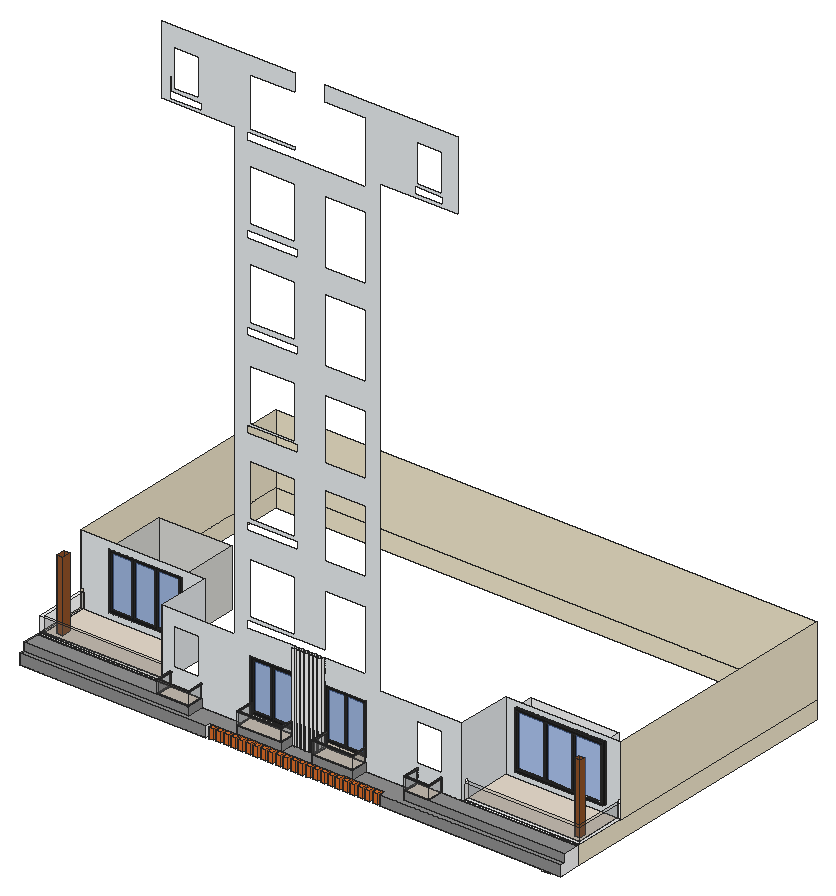
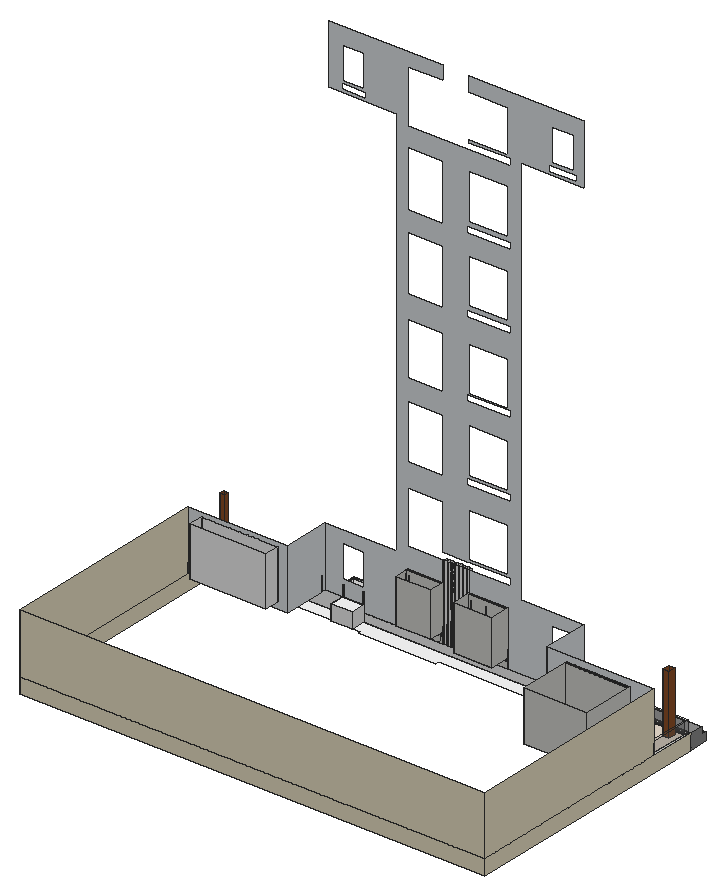
# SketchUp Ruby script. Lengths in inches.
U = 1.inch
M = Sketchup.active_model
def pt(a) = Geom::Point3d.new(a.map { |v| v * U })
def face(e, loops, mat)
  f = e.add_face(loops[0].map { |a| pt(a) })
  loops[1..].each { |l| e.add_face(l.map { |a| pt(a) }).erase! }
  f.material = f.back_material = mat if mat
  f
end
# faces: each face lists its corners as indices into pts; further lists are holes
def faces(e, pts, list, mat = nil) = list.each { |f| face(e, (f[0].is_a?(Array) ? f : [f]).map { |l| l.map { |i| pts[i] } }, mat) }
# xy, xz, yz: faces in a plane at the given z, y or x. An outline is a flat list of corners, or four numbers for a rectangle; further outlines are holes
def ring(l) = l.size == 4 ? [[l[0], l[1]], [l[2], l[1]], [l[2], l[3]], [l[0], l[3]]] : l.each_slice(2).to_a
def flat(e, list, mat, &to3) = list.each { |f| face(e, (f[0].is_a?(Array) ? f : [f]).map { |l| ring(l).map { |u, v| to3.(u, v) } }, mat) }
def xy(e, z, list, mat = nil) = flat(e, list, mat) { |x, y| [x, y, z] }
def xz(e, y, list, mat = nil) = flat(e, list, mat) { |x, z| [x, y, z] }
def yz(e, x, list, mat = nil) = flat(e, list, mat) { |y, z| [x, y, z] }
def lines(e, pts, list) = list.each { |a, b| e.add_line(pt(pts[a]), pt(pts[b])) }
# prism: a flat outline (further loops are holes) pulled along v
def prism(e, loops, v, mat = nil)
  f = face(e, loops, mat); d = Geom::Vector3d.new(v.map { |x| x * U })
  f.pushpull(f.normal.samedirection?(d) ? d.length : -d.length)
end
def box(e, o, s, mat = nil) = prism(e, [[o, [o[0] + s[0], o[1], o[2]], [o[0] + s[0], o[1] + s[1], o[2]], [o[0], o[1] + s[1], o[2]]]], [0, 0, s[2]], mat)
def at(x, y, z, deg = 0) = Geom::Transformation.translation(pt([x, y, z])) * Geom::Transformation.rotation(ORIGIN, Z_AXIS, deg.degrees)
def axes(o, x, y, z) = Geom::Transformation.new([*x, 0, *y, 0, *z, 0, *pt(o).to_a, 1])
def part(name) = M.definitions.add(name)
# library, detail: a bought-in or finely detailed component or shape, given as its bounding box
def library(name, o, s) = part(name).tap { |d| box(d.entities, o, s) }
def detail(e, o, s) = box(e.add_group.entities, o, s)
def put(e, d, t, mat = nil) = e.add_instance(d, t).tap { |i| i.material = mat if mat }
def group(e, t, mat = nil) = e.add_group.tap { |g| g.transformation = t; g.material = mat if mat }.entities
root = M.entities
M.materials.add("Generic").color = [146, 146, 146]
M.materials.add("Generic\#3").color = [226, 112, 41]
M.materials.add("Generic\#4").color = [237, 241, 244]
M.materials.add("Generic\#5").color = [249, 239, 211]
M.materials.add("Generic\#7").color = [232, 220, 205]
M.materials.add("[Color M00]").color = [255, 255, 255]
M.materials.add("[Color M06]").color = [86, 86, 86]
M.materials.add("[Color M08]").color = [30, 30, 30]
M.materials.add("[Translucent Glass Blue]1").color = [100, 149, 237]
M.materials["[Translucent Glass Blue]1"].alpha = 0.5
M.materials.add("[Translucent Glass Gray]").color = [119, 119, 119]
M.materials["[Translucent Glass Gray]"].alpha = 0.16
M.materials.add("[Wood Cherry Original]").color = [150, 85, 41]
M.materials.add("[Wood Cherry Original]1").color = [152, 86, 42]
c1 = part("Group\#10")
xy(c1.entities,0,[[0,0,98.1875,6]],"[Color M08]")
xy(c1.entities,5.79,[[5.79,0,46.2,3],[51.99,0,92.4,3]],"[Color M08]")
xy(c1.entities,117.02,[[5.79,0,46.2,3],[51.99,0,92.4,3]],"[Color M08]")
xy(c1.entities,122.8125,[[0,0,98.1875,6]],"[Color M08]")
xz(c1.entities,0,[[[0,0,98.1875,122.8125],[5.79,5.79,46.2,117.02],[51.99,5.79,92.4,117.02]]],"[Color M08]")
xz(c1.entities,3,[[5.79,5.79,46.2,117.02],[51.99,5.79,92.4,117.02]],"[Translucent Glass Blue]1")
xz(c1.entities,6,[[0,0,98.1875,122.8125]])
yz(c1.entities,0,[[0,0,6,122.8125]],"[Color M08]")
yz(c1.entities,5.79,[[0,5.79,3,117.02]],"[Color M08]")
yz(c1.entities,46.2,[[0,5.79,3,117.02]],"[Color M08]")
yz(c1.entities,51.99,[[0,5.79,3,117.02]],"[Color M08]")
yz(c1.entities,92.4,[[0,5.79,3,117.02]],"[Color M08]")
yz(c1.entities,98.1875,[[0,0,6,122.8125]],"[Color M08]")
c2 = part("Group\#11")
xy(c2.entities,0,[[0,0,175.8125,6]],"[Color M08]")
xy(c2.entities,7.33,[[7.33,0,56.16,3],[63.49,0,112.32,3],[119.65,0,168.48,3]],"[Color M08]")
xy(c2.entities,131.1,[[7.33,0,56.16,3],[63.49,0,112.32,3],[119.65,0,168.48,3]],"[Color M08]")
xy(c2.entities,138.4375,[[0,0,175.8125,6]],"[Color M08]")
xz(c2.entities,0,[[[0,0,175.8125,0,175.8125,131.1,168.48,131.1,168.48,7.33,119.65,7.33,119.65,131.1,175.8125,131.1,175.8125,138.4375,0,138.4375],[7.33,7.33,56.16,131.1],[63.49,7.33,112.32,131.1]]],"[Color M08]")
xz(c2.entities,3,[[7.33,7.33,56.16,131.1],[63.49,7.33,112.32,131.1],[119.65,7.33,168.48,131.1]],"[Translucent Glass Blue]1")
xz(c2.entities,6,[[0,0,175.8125,138.4375]])
yz(c2.entities,0,[[0,0,6,138.4375]],"[Color M08]")
yz(c2.entities,7.33,[[0,7.33,3,131.1]],"[Color M08]")
yz(c2.entities,56.16,[[0,7.33,3,131.1]],"[Color M08]")
yz(c2.entities,63.49,[[0,7.33,3,131.1]],"[Color M08]")
yz(c2.entities,112.32,[[0,7.33,3,131.1]],"[Color M08]")
yz(c2.entities,119.65,[[0,7.33,3,131.1]],"[Color M08]")
yz(c2.entities,168.48,[[0,7.33,3,131.1]],"[Color M08]")
yz(c2.entities,175.8125,[[0,0,6,138.4375]],"[Color M08]")
c3 = part("Group\#12")
xy(c3.entities,0,[[0,0,212.5625,7]],"[Color M08]")
xy(c3.entities,6.29,[[6.29,0,68.76,4],[75.05,0,137.52,4],[143.8,0,206.27,4]],"[Color M08]")
xy(c3.entities,131.21,[[6.29,0,68.76,4],[75.05,0,137.52,4],[143.8,0,206.27,4]],"[Color M08]")
xy(c3.entities,137.5,[[0,0,212.5625,7]],"[Color M08]")
xz(c3.entities,0,[[0,0,212.5625,6.29],[0,6.29,6.29,131.21],[68.76,6.29,75.05,131.21],[137.52,6.29,143.8,131.21],[206.27,6.29,212.5625,131.21],
  [0,131.21,212.5625,137.5]],"[Color M08]")
xz(c3.entities,4,[[6.29,6.29,68.76,131.21],[75.05,6.29,137.52,131.21],[143.8,6.29,206.27,131.21]],"[Translucent Glass Blue]1")
xz(c3.entities,7,[[0,0,212.5625,137.5]],"[Color M00]")
yz(c3.entities,0,[[0,0,7,137.5]],"[Color M08]")
yz(c3.entities,6.29,[[0,6.29,4,131.21]],"[Color M08]")
yz(c3.entities,68.76,[[0,6.29,4,131.21]],"[Color M08]")
yz(c3.entities,75.05,[[0,6.29,4,131.21]],"[Color M08]")
yz(c3.entities,137.52,[[0,6.29,4,131.21]],"[Color M08]")
yz(c3.entities,143.8,[[0,6.29,4,131.21]],"[Color M08]")
yz(c3.entities,206.27,[[0,6.29,4,131.21]],"[Color M08]")
yz(c3.entities,212.5625,[[0,0,7,137.5]],"[Color M08]")
xy(root,378.75,[[1471.55,257.9375,1493.05,261.625],[233.49,313.625,249.12,318.23]])
xy(root,378.75,[[209.5,261.625,209.5,313.625,233.49,313.625,233.49,296.48,249.12,296.48,249.12,313.625,509.5,313.625,509.5,261.625],[233.49,296.48,249.12,313.625]],"Generic")
xy(root,378.75,[[663.6,261.625,675.6,273.75],[681.6,261.625,693.6,273.75],[699.6,261.625,711.6,273.75],[717.6,261.625,729.6,273.75],[735.6,261.625,747.6,273.75],
  [753.6,261.625,765.6,273.75],[771.6,261.625,783.6,273.75],[789.6,261.625,801.6,273.75],[807.6,261.625,819.6,273.75],[825.6,261.625,837.6,273.75],
  [843.6,261.625,855.6,273.75],[861.6,261.625,873.6,273.75],[879.6,261.625,891.6,273.75],[897.6,261.625,909.6,273.75],[915.6,261.625,927.6,273.75],
  [933.6,261.625,945.6,273.75],[951.6,261.625,963.6,273.75],[969.6,261.625,981.6,273.75],[987.6,261.625,999.6,273.75],[1005.6,261.625,1017.6,273.75],
  [1023.6,261.625,1035.6,273.75],[1041.6,261.625,1053.6,273.75],[1059.6,261.625,1071.6,273.75]],"Generic\#3")
xy(root,378.75,[[509.5,261.625,509.5,313.625,1513,313.625,1513,261.625,1493.05,261.625,1493.05,285.22,1471.55,285.22,1471.55,261.625,1077.6,261.625,1077.6,273.75,657.6,273.75,657.6,261.625],[209.5,313.625,209.5,351.125,509.5,351.125,509.5,313.625,249.12,313.625,249.12,318.23,233.49,318.23,233.49,313.625],[509.5,313.625,509.5,360,548.8125,360,548.8125,351.125,886.67,351.125,886.67,360,1103.86,360,1103.86,351.125,1125.09,351.125,1125.09,313.625],[1125.09,313.625,1185.84,351.125],[1185.84,313.625,1513,351.125],
  [1125.09,351.125,1185.84,353.5]],"[Color M00]")
xy(root,403.0625,[[529.46,273.75,607.09,313.625],[722.84,273.75,830.21,313.625],[903.71,273.75,1001.9,313.625]])
xy(root,403.0625,[[209.5,261.625,657.6,261.625,657.6,273.75,722.84,273.75,722.84,313.625,607.09,313.625,607.09,273.75,209.5,273.75],[1077.6,261.625,1513,261.625,1513,273.75,1125.09,273.75,1125.09,313.625,1001.9,313.625,1001.9,273.75,1077.6,273.75],[830.21,273.75,903.71,273.75,903.71,313.625,901.15,313.625,901.15,305.3125,893.21,305.3125,893.21,313.625,890.65,313.625,890.65,305.3125,882.71,305.3125,882.71,313.625,880.15,313.625,880.15,305.3125,872.21,305.3125,872.21,313.625,869.65,313.625,869.65,305.3125,861.71,305.3125,861.71,313.625,859.15,313.625,859.15,305.3125,851.21,305.3125,851.21,313.625,848.65,313.625,848.65,305.3125,840.71,305.3125,840.71,313.625,838.15,313.625,838.15,305.3125,830.21,305.3125]],"Generic")
xy(root,403.0625,[[663.6,261.625,675.6,273.75],[681.6,261.625,693.6,273.75],[699.6,261.625,711.6,273.75],[717.6,261.625,729.6,273.75],[735.6,261.625,747.6,273.75],
  [753.6,261.625,765.6,273.75],[771.6,261.625,783.6,273.75],[789.6,261.625,801.6,273.75],[807.6,261.625,819.6,273.75],[825.6,261.625,837.6,273.75],
  [843.6,261.625,855.6,273.75],[861.6,261.625,873.6,273.75],[879.6,261.625,891.6,273.75],[897.6,261.625,909.6,273.75],[915.6,261.625,927.6,273.75],
  [933.6,261.625,945.6,273.75],[951.6,261.625,963.6,273.75],[969.6,261.625,981.6,273.75],[987.6,261.625,999.6,273.75],[1005.6,261.625,1017.6,273.75],
  [1023.6,261.625,1035.6,273.75],[1041.6,261.625,1053.6,273.75],[1059.6,261.625,1071.6,273.75]],"Generic\#3")
xy(root,403.0625,[[1125.09,273.75,1185.84,313.625],[830.21,305.3125,838.15,313.625],[840.71,305.3125,848.65,313.625],[851.21,305.3125,859.15,313.625],[861.71,305.3125,869.65,313.625],
  [872.21,305.3125,880.15,313.625],[882.71,305.3125,890.65,313.625],[893.21,305.3125,901.15,313.625]],"[Color M00]")
xy(root,421.5,[[529.46,273.75,532.46,313.625],[604.09,273.75,607.09,313.625],[722.84,273.75,830.21,276.75],[903.71,273.75,1001.9,276.75],[722.84,276.75,725.84,313.625],
  [827.21,276.75,830.21,313.625],[903.71,276.75,906.71,313.625],[998.9,276.75,1001.9,313.625],[209.5,313.625,509.5,320.625],[209.5,320.625,509.5,327.625],
  [209.5,327.625,216.5,444.3125],[234.12,340.02,249.74,361.77],[1483.76,340.63,1497.19,353.98]])
xy(root,421.5,[[209.5,273.75,529.46,313.625],[1185.84,273.75,1513,313.625]],"Generic")
xy(root,421.5,[[725.84,276.75,827.21,313.625],[906.71,276.75,998.9,313.625],[1128.09,276.75,1182.84,313.625],[532.46,276.9375,604.09,313.625],[[216.5,327.625,509.5,444.3125],[234.12,340.02,249.74,361.77]],
  [[1234.59,329.25,1506,444.3125],[1483.76,340.63,1497.19,353.98]]],"Generic\#7")
xy(root,421.5,[[1125.09,273.75,1185.84,276.75],[1125.09,276.75,1128.09,313.625],[1182.84,276.75,1185.84,313.625],[1125.09,313.625,1185.84,353.5],[1234.59,313.625,1513,320.625],
  [1234.59,320.625,1234.59,329.25,1506,329.25,1506,444.3125,1513,444.3125,1513,320.625]],"[Color M00]")
xy(root,421.5,[[532.46,273.75,604.09,276.9375]],"[Translucent Glass Gray]")
xy(root,429.75,[[722.84,313.625,830.21,367.5]])
xy(root,432.81,[[903.71,313.625,1001.9,356.375]])
xy(root,434.82,[[276.39,444.3125,452.2,595.9375]])
xy(root,439.82,[[1262.61,444.3125,1475.18,486.125]],"[Color M00]")
xy(root,451.5,[[529.46,273.75,529.46,313.625,532.46,313.625,532.46,276.9375,604.09,276.9375,604.09,313.625,607.09,313.625,607.09,273.75],[722.84,273.75,830.21,276.75],[903.71,273.75,1001.9,276.75],[722.84,276.75,725.84,313.625],[827.21,276.75,830.21,313.625],
  [903.71,276.75,906.71,313.625],[998.9,276.75,1001.9,313.625]])
xy(root,451.5,[[1125.09,273.75,1185.84,276.75],[1125.09,276.75,1128.09,313.625],[1182.84,276.75,1185.84,313.625]],"[Color M00]")
xz(root,261.625,[[209.5,378.75,657.6,403.0625],[1077.6,378.75,1513,403.0625]],"Generic")
xz(root,261.625,[[663.6,378.75,675.6,403.0625],[681.6,378.75,693.6,403.0625],[699.6,378.75,711.6,403.0625],[717.6,378.75,729.6,403.0625],[735.6,378.75,747.6,403.0625],
  [753.6,378.75,765.6,403.0625],[771.6,378.75,783.6,403.0625],[789.6,378.75,801.6,403.0625],[807.6,378.75,819.6,403.0625],[825.6,378.75,837.6,403.0625],
  [843.6,378.75,855.6,403.0625],[861.6,378.75,873.6,403.0625],[879.6,378.75,891.6,403.0625],[897.6,378.75,909.6,403.0625],[915.6,378.75,927.6,403.0625],
  [933.6,378.75,945.6,403.0625],[951.6,378.75,963.6,403.0625],[969.6,378.75,981.6,403.0625],[987.6,378.75,999.6,403.0625],[1005.6,378.75,1017.6,403.0625],
  [1023.6,378.75,1035.6,403.0625],[1041.6,378.75,1053.6,403.0625],[1059.6,378.75,1071.6,403.0625]],"Generic\#3")
xz(root,273.75,[[663.6,378.75,675.6,403.0625],[681.6,378.75,693.6,403.0625],[699.6,378.75,711.6,403.0625],[717.6,378.75,729.6,403.0625],[735.6,378.75,747.6,403.0625],
  [753.6,378.75,765.6,403.0625],[771.6,378.75,783.6,403.0625],[789.6,378.75,801.6,403.0625],[807.6,378.75,819.6,403.0625],[825.6,378.75,837.6,403.0625],
  [843.6,378.75,855.6,403.0625],[861.6,378.75,873.6,403.0625],[879.6,378.75,891.6,403.0625],[897.6,378.75,909.6,403.0625],[915.6,378.75,927.6,403.0625],
  [933.6,378.75,945.6,403.0625],[951.6,378.75,963.6,403.0625],[969.6,378.75,981.6,403.0625],[987.6,378.75,999.6,403.0625],[1005.6,378.75,1017.6,403.0625],
  [1023.6,378.75,1035.6,403.0625],[1041.6,378.75,1053.6,403.0625],[1059.6,378.75,1071.6,403.0625]])
xz(root,273.75,[[657.6,378.75,663.6,403.0625],[675.6,378.75,681.6,403.0625],[693.6,378.75,699.6,403.0625],[711.6,378.75,717.6,403.0625],[729.6,378.75,735.6,403.0625],
  [747.6,378.75,753.6,403.0625],[765.6,378.75,771.6,403.0625],[783.6,378.75,789.6,403.0625],[801.6,378.75,807.6,403.0625],[819.6,378.75,825.6,403.0625],
  [837.6,378.75,843.6,403.0625],[855.6,378.75,861.6,403.0625],[873.6,378.75,879.6,403.0625],[891.6,378.75,897.6,403.0625],[909.6,378.75,915.6,403.0625],
  [927.6,378.75,933.6,403.0625],[945.6,378.75,951.6,403.0625],[963.6,378.75,969.6,403.0625],[981.6,378.75,987.6,403.0625],[999.6,378.75,1005.6,403.0625],
  [1017.6,378.75,1023.6,403.0625],[1035.6,378.75,1041.6,403.0625],[1053.6,378.75,1059.6,403.0625],[1071.6,378.75,1077.6,403.0625],[209.5,403.0625,607.09,421.5],
  [722.84,403.0625,830.21,421.5],[903.71,403.0625,1001.9,421.5],[1125.09,403.0625,1513,421.5]],"Generic")
xz(root,273.75,[[529.46,451.5,607.09,454.25],[722.84,451.5,830.21,454.5],[903.71,451.5,1001.9,454.5],[1125.09,451.5,1185.84,454.5]],"[Color M06]")
xz(root,273.75,[[529.46,421.5,607.09,451.5],[722.84,421.5,830.21,451.5],[903.71,421.5,1001.9,451.5],[1125.09,421.5,1185.84,451.5]],"[Translucent Glass Gray]")
xz(root,276.75,[[725.84,451.5,827.21,454.5],[906.71,451.5,998.9,454.5]])
xz(root,276.75,[[1128.09,451.5,1182.84,454.5]],"[Color M00]")
xz(root,276.75,[[725.84,421.5,827.21,451.5],[906.71,421.5,998.9,451.5],[1128.09,421.5,1182.84,451.5]],"[Translucent Glass Gray]")
xz(root,276.9375,[[532.46,451.5,604.09,454.25]])
xz(root,276.9375,[[532.46,421.5,604.09,451.5]],"[Translucent Glass Gray]")
xz(root,305.3125,[[830.21,403.0625,838.15,613.8125],[840.71,403.0625,848.65,613.8125],[851.21,403.0625,859.15,613.8125],[861.71,403.0625,869.65,613.8125],[872.21,403.0625,880.15,613.8125],
  [882.71,403.0625,890.65,613.8125],[893.21,403.0625,901.15,613.8125]],"[Color M00]")
xz(root,313.625,[[529.46,403.0625,607.09,421.5],[722.84,403.0625,830.21,421.5],[903.71,403.0625,911.65,421.5],[911.65,403.0625,1001.9,421.5],[722.84,421.5,725.84,429.75],
  [725.84,421.5,827.21,429.75],[827.21,421.5,830.21,429.75],[903.71,421.5,906.71,432.81],[998.9,421.5,1001.9,432.81],[722.84,429.75,725.84,451.5],
  [827.21,429.75,830.21,451.5],[903.71,432.81,906.71,451.5],[998.9,432.81,1001.9,451.5],[722.84,451.5,725.84,454.5],[827.21,451.5,830.21,454.5],
  [903.71,451.5,906.71,454.5],[998.9,451.5,1001.9,454.5]])
xz(root,313.625,[[[607.09,403.0625,722.84,403.0625,722.84,555.62,830.21,555.62,830.21,613.8125,714.9,613.8125,714.9,665.25,717.9,665.25,717.9,632.25,835.15,632.25,835.15,665.25,838.15,665.25,838.15,632.25,903.71,632.25,903.71,758.4,1001.9,758.4,1001.9,613.8125,903.71,613.8125,903.71,555.62,1001.9,555.62,1001.9,403.0625,1125.09,403.0625,1125.09,454.5,1128.09,454.5,1128.09,421.5,1182.84,421.5,1182.84,454.5,1185.84,454.5,1185.84,421.5,1234.59,421.5,1234.59,589.5,1034.5,589.5,1034.5,1686,1224.95,1686,1224.95,1854,903.71,1854,903.71,1816.73,1001.9,1816.73,1001.9,1667.5625,714.9,1667.5625,714.9,1719,717.9,1719,717.9,1686,830.21,1686,830.21,1693.55,722.84,1693.55,722.84,1811.98,830.21,1811.98,830.21,1854,509.5,1854,509.5,1686,685.0625,1686,685.0625,589.5,509.5,589.5,509.5,421.5,529.46,421.5,529.46,454.25,532.46,454.25,532.46,421.5,604.09,421.5,604.09,454.25,607.09,454.25],[714.9,1035.3125,714.9,1086.75,717.9,1086.75,717.9,1053.75,830.21,1053.75,830.21,1056.17,722.84,1056.17,722.84,1182.05,830.21,1182.05,830.21,1053.75,835.15,1053.75,835.15,1086.75,838.15,1086.75,838.15,1035.3125],[903.71,1456.8125,1001.9,1613.9],[903.71,1246.0625,1001.9,1401.52],[903.71,824.5625,1001.9,976.4],[903.71,1035.3125,1001.9,1182.15],[722.84,1275.65,830.21,1401.52],[722.84,850.52,830.21,976.4],[722.84,638.46,830.21,764.34],[722.84,1488.02,830.21,1613.9],[1120.78,1693.68,1120.78,1743.93,1122.9,1743.93,1122.9,1710.93,1185.6,1710.93,1185.6,1716.73,1125.09,1716.73,1125.09,1806.86,1185.84,1806.86,1185.84,1743.93,1188.6,1743.93,1188.6,1693.68],[537.9,1716.73,598.65,1806.86],[1125.09,465.5,1185.84,555.62],[537.9,465.5,598.65,555.62],[714.9,1456.8125,714.9,1508.25,717.9,1508.25,717.9,1475.25,835.15,1475.25,835.15,1508.25,838.15,1508.25,838.15,1456.8125],[714.9,824.5625,714.9,876,717.9,876,717.9,843,835.15,843,835.15,876,838.15,876,838.15,824.5625],[714.9,1246.0625,714.9,1297.5,717.9,1297.5,717.9,1264.5,835.15,1264.5,835.15,1297.5,838.15,1297.5,838.15,1246.0625],[529.46,1691.95,529.46,1742.5,532.46,1742.5,532.46,1709.75,604.09,1709.75,604.09,1742.5,607.09,1742.5,607.09,1691.95],[1185.6,1716.73,1185.84,1743.93]]],"Generic\#4")
xz(root,313.625,[[906.71,421.5,998.9,432.81]],"Generic\#7")
xz(root,313.625,[[209.5,378.75,209.5,421.5,529.46,421.5,529.46,403.0625,509.5,403.0625,509.5,378.75],[509.5,378.75,1125.09,403.0625],[1125.09,378.75,1185.84,403.0625],[1185.84,378.75,1513,421.5],[830.21,403.0625,838.15,613.8125],
  [838.15,403.0625,840.71,613.8125],[840.71,403.0625,848.65,613.8125],[848.65,403.0625,851.21,613.8125],[851.21,403.0625,859.15,613.8125],[859.15,403.0625,861.71,613.8125],
  [861.71,403.0625,869.65,613.8125],[869.65,403.0625,872.21,613.8125],[872.21,403.0625,880.15,613.8125],[880.15,403.0625,882.71,613.8125],[882.71,403.0625,890.65,613.8125],
  [890.65,403.0625,893.21,613.8125],[893.21,403.0625,901.15,613.8125],[901.15,403.0625,903.71,613.8125],[1125.09,403.0625,1185.84,421.5],[1125.09,421.5,1128.09,451.5],
  [1182.84,421.5,1185.84,451.5],[1125.09,451.5,1128.09,454.5],[1182.84,451.5,1185.84,454.5]],"[Color M00]")
xz(root,320.625,[[209.5,421.5,509.5,457.5],[1234.59,421.5,1513,457.5]],"[Translucent Glass Gray]")
xz(root,327.625,[[216.5,421.5,509.5,457.5]],"[Translucent Glass Gray]")
xz(root,329.25,[[1234.59,421.5,1506,457.5]],"[Translucent Glass Gray]")
xz(root,340.02,[[234.12,421.5,249.74,589.5]],"[Wood Cherry Original]1")
xz(root,340.63,[[1483.76,421.5,1497.19,589.5]],"[Wood Cherry Original]")
xz(root,353.5,[[1125.09,378.75,1185.84,421.5]],"[Color M00]")
xz(root,353.98,[[1483.76,421.5,1497.19,589.5]],"[Wood Cherry Original]")
xz(root,356.375,[[903.71,432.81,1001.9,555.62]])
xz(root,361.77,[[234.12,421.5,249.74,589.5]],"[Wood Cherry Original]1")
xz(root,367.5,[[722.84,429.75,830.21,555.62]])
xz(root,444.3125,[[209.5,421.5,216.5,457.5]])
xz(root,444.3125,[[[216.5,421.5,509.5,421.5,509.5,589.5,209.5,589.5,209.5,464.5,216.5,464.5],[276.39,434.82,452.2,573.26]],[[1234.59,421.5,1506,421.5,1506,463.9375,1513,463.9375,1513,589.5,1234.59,589.5],[1262.61,439.82,1475.18,577.32]]],"Generic\#4")
xz(root,486.125,[[1262.61,439.82,1475.18,577.32]],"[Color M00]")
xz(root,595.9375,[[276.39,434.82,452.2,573.26]])
xz(root,1033.625,[[209.5,378.75,1513,421.5],[209.5,421.5,1513,589.5]],"Generic\#5")
yz(root,209.5,[[261.625,378.75,261.625,403.0625,273.75,403.0625,273.75,421.5,313.625,421.5,313.625,378.75]],"Generic")
yz(root,209.5,[[313.625,378.75,1033.625,421.5],[444.3125,421.5,1033.625,589.5]],"Generic\#5")
yz(root,209.5,[[320.625,421.5,444.3125,457.5]],"[Translucent Glass Gray]")
yz(root,216.5,[[327.625,421.5,444.3125,457.5]],"[Translucent Glass Gray]")
yz(root,234.12,[[340.02,421.5,361.77,589.5]],"[Wood Cherry Original]1")
yz(root,249.74,[[340.02,421.5,361.77,589.5]],"[Wood Cherry Original]1")
yz(root,276.39,[[444.3125,434.82,595.9375,573.26]])
yz(root,452.2,[[444.3125,434.82,595.9375,573.26]])
yz(root,509.5,[[320.625,421.5,327.625,457.5]])
yz(root,509.5,[[313.625,421.5,313.625,589.5,444.3125,589.5,444.3125,421.5,327.625,421.5,327.625,464.5,320.625,464.5,320.625,421.5]],"Generic\#4")
yz(root,529.46,[[273.75,451.5,313.625,454.25]],"[Color M06]")
yz(root,529.46,[[273.75,421.5,313.625,451.5]],"[Translucent Glass Gray]")
yz(root,532.46,[[276.9375,451.5,313.625,454.25]],"[Color M06]")
yz(root,532.46,[[276.9375,421.5,313.625,451.5]],"[Translucent Glass Gray]")
yz(root,604.09,[[276.9375,451.5,313.625,454.25]],"[Color M06]")
yz(root,604.09,[[276.9375,421.5,313.625,451.5]],"[Translucent Glass Gray]")
yz(root,607.09,[[273.75,403.0625,313.625,421.5]],"Generic")
yz(root,607.09,[[273.75,451.5,313.625,454.25]],"[Color M06]")
yz(root,607.09,[[273.75,421.5,313.625,451.5]],"[Translucent Glass Gray]")
yz(root,657.6,[[261.625,378.75,273.75,403.0625]],"[Color M00]")
yz(root,663.6,[[261.625,378.75,273.75,403.0625]],"Generic\#3")
yz(root,675.6,[[261.625,378.75,273.75,403.0625]],"Generic\#3")
yz(root,681.6,[[261.625,378.75,273.75,403.0625]],"Generic\#3")
yz(root,693.6,[[261.625,378.75,273.75,403.0625]],"Generic\#3")
yz(root,699.6,[[261.625,378.75,273.75,403.0625]],"Generic\#3")
yz(root,711.6,[[261.625,378.75,273.75,403.0625]],"Generic\#3")
yz(root,717.6,[[261.625,378.75,273.75,403.0625]],"Generic\#3")
yz(root,722.84,[[313.625,429.75,367.5,555.62]])
yz(root,722.84,[[273.75,403.0625,313.625,421.5]],"Generic")
yz(root,722.84,[[273.75,451.5,313.625,454.5]],"[Color M06]")
yz(root,722.84,[[273.75,421.5,313.625,451.5]],"[Translucent Glass Gray]")
yz(root,725.84,[[276.75,451.5,313.625,454.5]],"[Color M06]")
yz(root,725.84,[[276.75,421.5,313.625,451.5]],"[Translucent Glass Gray]")
yz(root,729.6,[[261.625,378.75,273.75,403.0625]],"Generic\#3")
yz(root,735.6,[[261.625,378.75,273.75,403.0625]],"Generic\#3")
yz(root,747.6,[[261.625,378.75,273.75,403.0625]],"Generic\#3")
yz(root,753.6,[[261.625,378.75,273.75,403.0625]],"Generic\#3")
yz(root,765.6,[[261.625,378.75,273.75,403.0625]],"Generic\#3")
yz(root,771.6,[[261.625,378.75,273.75,403.0625]],"Generic\#3")
yz(root,783.6,[[261.625,378.75,273.75,403.0625]],"Generic\#3")
yz(root,789.6,[[261.625,378.75,273.75,403.0625]],"Generic\#3")
yz(root,801.6,[[261.625,378.75,273.75,403.0625]],"Generic\#3")
yz(root,807.6,[[261.625,378.75,273.75,403.0625]],"Generic\#3")
yz(root,819.6,[[261.625,378.75,273.75,403.0625]],"Generic\#3")
yz(root,825.6,[[261.625,378.75,273.75,403.0625]],"Generic\#3")
yz(root,827.21,[[276.75,451.5,313.625,454.5]],"[Color M06]")
yz(root,827.21,[[276.75,421.5,313.625,451.5]],"[Translucent Glass Gray]")
yz(root,830.21,[[313.625,429.75,367.5,555.62]])
yz(root,830.21,[[273.75,403.0625,305.3125,421.5]],"Generic")
yz(root,830.21,[[305.3125,403.0625,313.625,421.5],[305.3125,421.5,313.625,429.75],[305.3125,429.75,313.625,451.5],[305.3125,451.5,313.625,454.5]],"[Color M00]")
yz(root,830.21,[[273.75,451.5,305.3125,454.5]],"[Color M06]")
yz(root,830.21,[[273.75,421.5,305.3125,451.5]],"[Translucent Glass Gray]")
yz(root,837.6,[[261.625,378.75,273.75,403.0625]],"Generic\#3")
yz(root,838.15,[[305.3125,403.0625,313.625,613.8125]],"[Color M00]")
yz(root,840.71,[[305.3125,403.0625,313.625,421.5],[305.3125,421.5,313.625,429.75],[305.3125,429.75,313.625,451.5],[305.3125,451.5,313.625,454.5]],"[Color M00]")
yz(root,843.6,[[261.625,378.75,273.75,403.0625]],"Generic\#3")
yz(root,848.65,[[305.3125,403.0625,313.625,613.8125]],"[Color M00]")
yz(root,851.21,[[305.3125,403.0625,313.625,421.5],[305.3125,421.5,313.625,429.75],[305.3125,429.75,313.625,451.5],[305.3125,451.5,313.625,454.5]],"[Color M00]")
yz(root,855.6,[[261.625,378.75,273.75,403.0625]],"Generic\#3")
yz(root,859.15,[[305.3125,403.0625,313.625,613.8125]],"[Color M00]")
yz(root,861.6,[[261.625,378.75,273.75,403.0625]],"Generic\#3")
yz(root,861.71,[[305.3125,403.0625,313.625,421.5],[305.3125,421.5,313.625,429.75],[305.3125,429.75,313.625,451.5],[305.3125,451.5,313.625,454.5]],"[Color M00]")
yz(root,869.65,[[305.3125,403.0625,313.625,613.8125]],"[Color M00]")
yz(root,872.21,[[305.3125,403.0625,313.625,421.5],[305.3125,421.5,313.625,429.75],[305.3125,429.75,313.625,451.5],[305.3125,451.5,313.625,454.5]],"[Color M00]")
yz(root,873.6,[[261.625,378.75,273.75,403.0625]],"Generic\#3")
yz(root,879.6,[[261.625,378.75,273.75,403.0625]],"Generic\#3")
yz(root,880.15,[[305.3125,403.0625,313.625,613.8125]],"[Color M00]")
yz(root,882.71,[[305.3125,403.0625,313.625,421.5],[305.3125,421.5,313.625,429.75],[305.3125,429.75,313.625,451.5],[305.3125,451.5,313.625,454.5]],"[Color M00]")
yz(root,890.65,[[305.3125,403.0625,313.625,613.8125]],"[Color M00]")
yz(root,891.6,[[261.625,378.75,273.75,403.0625]],"Generic\#3")
yz(root,893.21,[[305.3125,403.0625,313.625,421.5],[305.3125,421.5,313.625,429.75],[305.3125,429.75,313.625,451.5],[305.3125,451.5,313.625,454.5]],"[Color M00]")
yz(root,897.6,[[261.625,378.75,273.75,403.0625]],"Generic\#3")
yz(root,901.15,[[305.3125,403.0625,313.625,613.8125]],"[Color M00]")
yz(root,903.71,[[313.625,432.81,356.375,555.62]])
yz(root,903.71,[[273.75,403.0625,313.625,421.5]],"Generic")
yz(root,903.71,[[273.75,451.5,313.625,454.5]],"[Color M06]")
yz(root,903.71,[[273.75,421.5,313.625,451.5]],"[Translucent Glass Gray]")
yz(root,906.71,[[276.75,451.5,313.625,454.5]],"[Color M06]")
yz(root,906.71,[[276.75,421.5,313.625,451.5]],"[Translucent Glass Gray]")
yz(root,909.6,[[261.625,378.75,273.75,403.0625]],"Generic\#3")
yz(root,915.6,[[261.625,378.75,273.75,403.0625]],"Generic\#3")
yz(root,927.6,[[261.625,378.75,273.75,403.0625]],"Generic\#3")
yz(root,933.6,[[261.625,378.75,273.75,403.0625]],"Generic\#3")
yz(root,945.6,[[261.625,378.75,273.75,403.0625]],"Generic\#3")
yz(root,951.6,[[261.625,378.75,273.75,403.0625]],"Generic\#3")
yz(root,963.6,[[261.625,378.75,273.75,403.0625]],"Generic\#3")
yz(root,969.6,[[261.625,378.75,273.75,403.0625]],"Generic\#3")
yz(root,981.6,[[261.625,378.75,273.75,403.0625]],"Generic\#3")
yz(root,987.6,[[261.625,378.75,273.75,403.0625]],"Generic\#3")
yz(root,998.9,[[276.75,451.5,313.625,454.5]],"[Color M06]")
yz(root,998.9,[[276.75,421.5,313.625,451.5]],"[Translucent Glass Gray]")
yz(root,999.6,[[261.625,378.75,273.75,403.0625]],"Generic\#3")
yz(root,1001.9,[[313.625,432.81,356.375,555.62]])
yz(root,1001.9,[[273.75,403.0625,313.625,421.5]],"Generic")
yz(root,1001.9,[[273.75,451.5,313.625,454.5]],"[Color M06]")
yz(root,1001.9,[[273.75,421.5,313.625,451.5]],"[Translucent Glass Gray]")
yz(root,1005.6,[[261.625,378.75,273.75,403.0625]],"Generic\#3")
yz(root,1017.6,[[261.625,378.75,273.75,403.0625]],"Generic\#3")
yz(root,1023.6,[[261.625,378.75,273.75,403.0625]],"Generic\#3")
yz(root,1035.6,[[261.625,378.75,273.75,403.0625]],"Generic\#3")
yz(root,1041.6,[[261.625,378.75,273.75,403.0625]],"Generic\#3")
yz(root,1053.6,[[261.625,378.75,273.75,403.0625]],"Generic\#3")
yz(root,1059.6,[[261.625,378.75,273.75,403.0625]],"Generic\#3")
yz(root,1071.6,[[261.625,378.75,273.75,403.0625]],"Generic\#3")
yz(root,1077.6,[[261.625,378.75,273.75,403.0625]],"Generic\#3")
yz(root,1125.09,[[273.75,403.0625,313.625,421.5]],"Generic")
yz(root,1125.09,[[313.625,378.75,353.5,421.5]],"[Color M00]")
yz(root,1125.09,[[273.75,451.5,313.625,454.5]],"[Color M06]")
yz(root,1125.09,[[273.75,421.5,313.625,451.5]],"[Translucent Glass Gray]")
yz(root,1128.09,[[276.75,451.5,313.625,454.5]],"[Color M06]")
yz(root,1128.09,[[276.75,421.5,313.625,451.5]],"[Translucent Glass Gray]")
yz(root,1182.84,[[276.75,451.5,313.625,454.5]],"[Color M06]")
yz(root,1182.84,[[276.75,421.5,313.625,451.5]],"[Translucent Glass Gray]")
yz(root,1185.84,[[313.625,378.75,353.5,421.5]],"[Color M00]")
yz(root,1185.84,[[273.75,451.5,313.625,454.5]],"[Color M06]")
yz(root,1185.84,[[273.75,421.5,313.625,451.5]],"[Translucent Glass Gray]")
yz(root,1234.59,[[313.625,421.5,320.625,421.5,320.625,463.9375,329.25,463.9375,329.25,421.5,444.3125,421.5,444.3125,589.5,313.625,589.5]],"Generic\#4")
yz(root,1234.59,[[320.625,421.5,329.25,457.5]],"[Color M00]")
yz(root,1262.61,[[444.3125,439.82,486.125,577.32]],"[Color M00]")
yz(root,1475.18,[[444.3125,439.82,486.125,577.32]],"[Color M00]")
yz(root,1483.76,[[340.63,421.5,353.98,589.5]],"[Wood Cherry Original]")
yz(root,1497.19,[[340.63,421.5,353.98,589.5]],"[Wood Cherry Original]")
yz(root,1506,[[329.25,421.5,444.3125,457.5]],"[Translucent Glass Gray]")
yz(root,1513,[[313.625,378.75,1033.625,421.5],[444.3125,421.5,1033.625,589.5]],"Generic\#5")
yz(root,1513,[[261.625,378.75,313.625,378.75,313.625,421.5,273.75,421.5,273.75,403.0625,261.625,403.0625]],"[Color M00]")
yz(root,1513,[[320.625,421.5,444.3125,457.5]],"[Translucent Glass Gray]")
g1 = group(root,at(722.84,313.625,429.75))
xy(g1,0,[[0,0,107.375,6]],"[Color M08]")
xy(g1,7.85,[[7.85,0,49.76,3],[57.61,0,99.52,3]],"[Color M08]")
xy(g1,118.02,[[7.85,0,49.76,3],[57.61,0,99.52,3]],"[Color M08]")
xy(g1,125.875,[[0,0,107.375,6]],"[Color M08]")
xz(g1,0,[[[0,0,107.375,125.875],[57.61,7.85,99.52,118.02],[7.85,7.85,49.76,118.02]]],"[Color M08]")
xz(g1,3,[[7.85,7.85,49.76,118.02],[57.61,7.85,99.52,118.02]],"[Translucent Glass Blue]1")
xz(g1,6,[[0,0,107.375,125.875]])
yz(g1,0,[[0,0,6,125.875]],"[Color M08]")
yz(g1,7.85,[[0,7.85,3,118.02]],"[Color M08]")
yz(g1,49.76,[[0,7.85,3,118.02]],"[Color M08]")
yz(g1,57.61,[[0,7.85,3,118.02]],"[Color M08]")
yz(g1,99.52,[[0,7.85,3,118.02]],"[Color M08]")
yz(g1,107.375,[[0,0,6,125.875]],"[Color M08]")
put(root,c1,at(903.71,313.625,432.81))
put(root,c2,at(276.39,444.3125,434.82))
put(root,c3,at(1262.61,437.3125,439.82))
